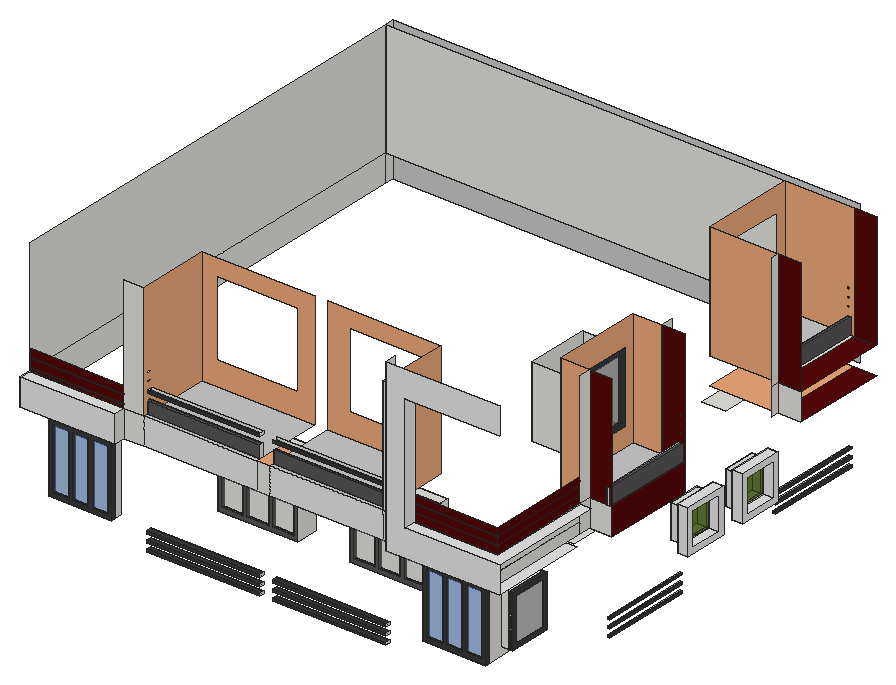
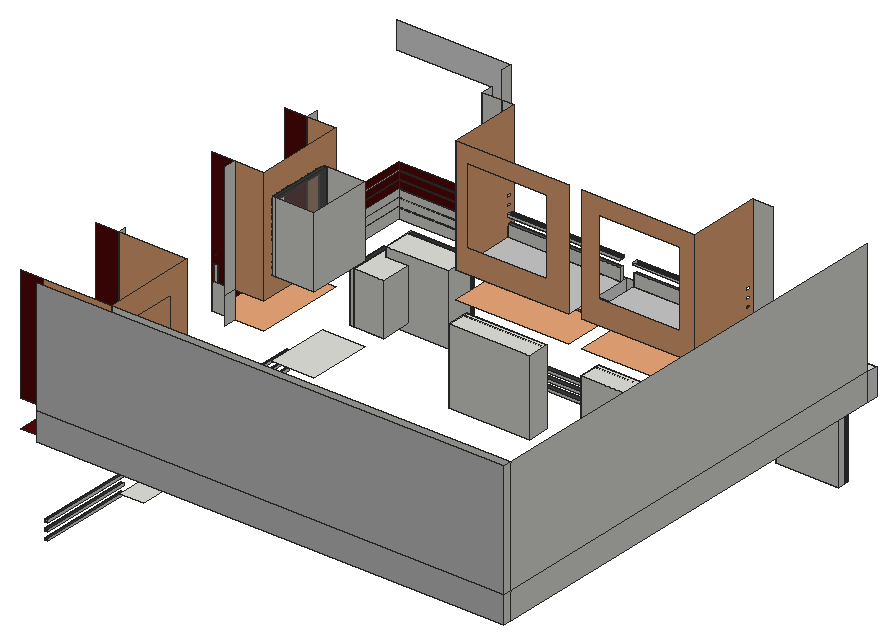
# SketchUp Ruby script. Lengths in inches.
U = 1.inch
M = Sketchup.active_model
def pt(a) = Geom::Point3d.new(a.map { |v| v * U })
def face(e, loops, mat)
  f = e.add_face(loops[0].map { |a| pt(a) })
  loops[1..].each { |l| e.add_face(l.map { |a| pt(a) }).erase! }
  f.material = f.back_material = mat if mat
  f
end
# faces: each face lists its corners as indices into pts; further lists are holes
def faces(e, pts, list, mat = nil) = list.each { |f| face(e, (f[0].is_a?(Array) ? f : [f]).map { |l| l.map { |i| pts[i] } }, mat) }
# xy, xz, yz: faces in a plane at the given z, y or x. An outline is a flat list of corners, or four numbers for a rectangle; further outlines are holes
def ring(l) = l.size == 4 ? [[l[0], l[1]], [l[2], l[1]], [l[2], l[3]], [l[0], l[3]]] : l.each_slice(2).to_a
def flat(e, list, mat, &to3) = list.each { |f| face(e, (f[0].is_a?(Array) ? f : [f]).map { |l| ring(l).map { |u, v| to3.(u, v) } }, mat) }
def xy(e, z, list, mat = nil) = flat(e, list, mat) { |x, y| [x, y, z] }
def xz(e, y, list, mat = nil) = flat(e, list, mat) { |x, z| [x, y, z] }
def yz(e, x, list, mat = nil) = flat(e, list, mat) { |y, z| [x, y, z] }
def lines(e, pts, list) = list.each { |a, b| e.add_line(pt(pts[a]), pt(pts[b])) }
# prism: a flat outline (further loops are holes) pulled along v
def prism(e, loops, v, mat = nil)
  f = face(e, loops, mat); d = Geom::Vector3d.new(v.map { |x| x * U })
  f.pushpull(f.normal.samedirection?(d) ? d.length : -d.length)
end
def box(e, o, s, mat = nil) = prism(e, [[o, [o[0] + s[0], o[1], o[2]], [o[0] + s[0], o[1] + s[1], o[2]], [o[0], o[1] + s[1], o[2]]]], [0, 0, s[2]], mat)
def at(x, y, z, deg = 0) = Geom::Transformation.translation(pt([x, y, z])) * Geom::Transformation.rotation(ORIGIN, Z_AXIS, deg.degrees)
def axes(o, x, y, z) = Geom::Transformation.new([*x, 0, *y, 0, *z, 0, *pt(o).to_a, 1])
def part(name) = M.definitions.add(name)
# library, detail: a bought-in or finely detailed component or shape, given as its bounding box
def library(name, o, s) = part(name).tap { |d| box(d.entities, o, s) }
def detail(e, o, s) = box(e.add_group.entities, o, s)
def put(e, d, t, mat = nil) = e.add_instance(d, t).tap { |i| i.material = mat if mat }
def group(e, t, mat = nil) = e.add_group.tap { |g| g.transformation = t; g.material = mat if mat }.entities
root = M.entities
M.materials.add("Generic").color = [86, 8, 8]
M.materials.add("Generic\#1").color = [236, 168, 122]
M.materials.add("Generic\#4").color = [201, 201, 201]
M.materials.add("Generic\#5").color = [230, 230, 230]
M.materials.add("[Color M06]").color = [86, 86, 86]
M.materials.add("[Color M07]").color = [58, 58, 58]
M.materials.add("[Mirror 01]").color = [185, 185, 185]
M.materials.add("[Mirror 02]1").color = [226, 226, 226]
M.materials["[Mirror 02]1"].alpha = 0.26
M.materials.add("[Translucent Glass Blue]").color = [100, 149, 237]
M.materials["[Translucent Glass Blue]"].alpha = 0.5
M.materials.add("[Translucent Glass Dark Green]").color = [62, 91, 5]
M.materials["[Translucent Glass Dark Green]"].alpha = 0.5
M.materials.add("[Translucent Glass Gray]").color = [127, 127, 127]
M.materials["[Translucent Glass Gray]"].alpha = 0.35
c1 = part("Group\#4")
xy(c1.entities,0,[[0,0,117.75,6]],"[Color M06]")
xy(c1.entities,6.37,[[6.37,0,37.125,3],[43.5,0,74.25,3],[80.625,0,111.38,3]],"[Color M06]")
xy(c1.entities,103.75,[[6.37,0,37.125,3],[43.5,0,74.25,3],[80.625,0,111.38,3]],"[Color M06]")
xy(c1.entities,110.125,[[0,0,117.75,6]],"[Color M06]")
xz(c1.entities,0,[[[0,0,117.75,110.125],[6.37,6.37,37.125,103.75],[80.625,6.37,111.38,103.75],[43.5,6.37,74.25,103.75]]],"[Color M06]")
xz(c1.entities,3,[[6.37,6.37,37.125,103.75],[43.5,6.37,74.25,103.75],[80.625,6.37,111.38,103.75]],"[Mirror 02]1")
xz(c1.entities,6,[[0,0,117.75,110.125]])
yz(c1.entities,0,[[0,0,6,110.125]],"[Color M06]")
yz(c1.entities,6.37,[[0,6.37,3,103.75]],"[Color M06]")
yz(c1.entities,37.125,[[0,6.37,3,103.75]],"[Color M06]")
yz(c1.entities,43.5,[[0,6.37,3,103.75]],"[Color M06]")
yz(c1.entities,74.25,[[0,6.37,3,103.75]],"[Color M06]")
yz(c1.entities,80.625,[[0,6.37,3,103.75]],"[Color M06]")
yz(c1.entities,111.38,[[0,6.37,3,103.75]],"[Color M06]")
yz(c1.entities,117.75,[[0,0,6,110.125]],"[Color M06]")
c2 = part("Group\#2")
xy(c2.entities,0,[[0,0,91.6875,6]],"[Color M07]")
xy(c2.entities,6.1,[[6.1,0,28.53,3],[34.63,0,57.06,3],[63.16,0,85.59,3]],"[Color M07]")
xy(c2.entities,95.34,[[6.1,0,28.53,3],[34.63,0,57.06,3],[63.16,0,85.59,3]],"[Color M07]")
xy(c2.entities,101.4375,[[0,0,91.6875,6]],"[Color M07]")
xz(c2.entities,0,[[[0,0,91.6875,101.4375],[34.63,6.1,57.06,95.34],[63.16,6.1,85.59,95.34],[6.1,6.1,28.53,95.34]]],"[Color M07]")
xz(c2.entities,3,[[6.1,6.1,28.53,95.34],[34.63,6.1,57.06,95.34],[63.16,6.1,85.59,95.34]],"[Translucent Glass Blue]")
xz(c2.entities,6,[[0,0,91.6875,101.4375]])
yz(c2.entities,0,[[0,0,6,101.4375]],"[Color M07]")
yz(c2.entities,6.1,[[0,6.1,3,95.34]],"[Color M07]")
yz(c2.entities,28.53,[[0,6.1,3,95.34]],"[Color M07]")
yz(c2.entities,34.63,[[0,6.1,3,95.34]],"[Color M07]")
yz(c2.entities,57.06,[[0,6.1,3,95.34]],"[Color M07]")
yz(c2.entities,63.16,[[0,6.1,3,95.34]],"[Color M07]")
yz(c2.entities,85.59,[[0,6.1,3,95.34]],"[Color M07]")
yz(c2.entities,91.6875,[[0,0,6,101.4375]],"[Color M07]")
c3 = part("Group\#3")
xy(c3.entities,0,[[0,0,6,62.6875]],"[Color M07]")
xy(c3.entities,6.1,[[3,6.1,6,56.59]],"[Color M07]")
xy(c3.entities,69.52,[[3,6.1,6,56.59]],"[Color M07]")
xy(c3.entities,75.625,[[0,0,6,62.6875]],"[Color M07]")
xz(c3.entities,0,[[0,0,6,75.625]],"[Color M07]")
xz(c3.entities,6.1,[[3,6.1,6,69.52]],"[Color M07]")
xz(c3.entities,56.59,[[3,6.1,6,69.52]],"[Color M07]")
xz(c3.entities,62.6875,[[0,0,6,75.625]],"[Color M07]")
yz(c3.entities,0,[[0,0,62.6875,75.625]])
yz(c3.entities,3,[[6.1,6.1,56.59,69.52]],"[Mirror 01]")
yz(c3.entities,6,[[[0,0,62.6875,75.625],[6.1,6.1,56.59,69.52]]],"[Color M07]")
c4 = part("Group\#1")
box(c4.entities,[0,0,0],[3,48.3125,48.3125],"[Translucent Glass Dark Green]")
c5 = library("Tlon Light 450 Ceiling 152 006",[-8.86,-8.86,-3.78],[17.72,17.72,3.56])
c6 = part("Group\#5")
xy(c6.entities,0,[[0,0,6,92.0625]],"[Color M07]")
xy(c6.entities,6.58,[[3,6.58,6,85.48]],"[Color M07]")
xy(c6.entities,96.73,[[3,6.58,6,85.48]],"[Color M07]")
xy(c6.entities,103.3125,[[0,0,6,92.0625]],"[Color M07]")
xz(c6.entities,0,[[0,0,6,103.3125]],"[Color M07]")
xz(c6.entities,6.58,[[3,6.58,6,96.73]],"[Color M07]")
xz(c6.entities,85.48,[[3,6.58,6,96.73]],"[Color M07]")
xz(c6.entities,92.0625,[[0,0,6,103.3125]],"[Color M07]")
yz(c6.entities,0,[[0,0,92.0625,103.3125]],"[Translucent Glass Gray]")
yz(c6.entities,3,[[6.58,6.58,85.48,96.73]],"[Translucent Glass Gray]")
yz(c6.entities,6,[[[0,0,92.0625,103.3125],[6.58,6.58,85.48,96.73]]],"[Color M07]")
xy(root,442.38,[[183.5625,118.5,347.9375,125.9375]],"[Color M07]")
xy(root,442.82,[[367.1875,118.5,531.5625,125.9375]],"[Color M07]")
xy(root,446.19,[[183.5625,118.5,347.9375,125.9375]],"[Color M07]")
xy(root,446.63,[[367.1875,118.5,531.5625,125.9375]],"[Color M07]")
xy(root,449.49,[[691.43,624.8125,695.61,762.8125]],"[Color M07]")
xy(root,449.67,[[724.45,281.625,727.82,413.625]],"[Color M07]")
xy(root,452.79,[[724.45,281.625,727.82,413.625]],"[Color M07]")
xy(root,452.8,[[691.43,624.8125,695.61,762.8125]],"[Color M07]")
xy(root,454.38,[[183.5625,118.5,347.9375,125.9375]],"[Color M07]")
xy(root,454.82,[[367.1875,118.5,531.5625,125.9375]],"[Color M07]")
xy(root,458.19,[[183.5625,118.5,347.9375,125.9375]],"[Color M07]")
xy(root,458.63,[[367.1875,118.5,531.5625,125.9375]],"[Color M07]")
xy(root,460.21,[[205.67,219.4375,323.42,251.5625],[397.99,219.4375,515.74,251.5625]])
xy(root,461.54,[[691.43,624.8125,695.61,762.8125]],"[Color M07]")
xy(root,461.67,[[724.45,281.625,727.82,413.625]],"[Color M07]")
xy(root,464.79,[[724.45,281.625,727.82,413.625]],"[Color M07]")
xy(root,464.85,[[691.43,624.8125,695.61,762.8125]],"[Color M07]")
xy(root,466.73,[[183.5625,118.5,347.9375,125.9375]],"[Color M07]")
xy(root,466.82,[[367.1875,118.5,531.5625,125.9375]],"[Color M07]")
xy(root,468.8,[[44.83,113.625,136.51,130.0625]])
xy(root,470.54,[[183.5625,118.5,347.9375,125.9375]],"[Color M07]")
xy(root,470.63,[[367.1875,118.5,531.5625,125.9375]],"[Color M07]")
xy(root,471.43,[[589.83,113.625,681.51,159.375]])
xy(root,473.54,[[691.43,624.8125,695.61,762.8125]],"[Color M07]")
xy(root,473.55,[[724.45,281.625,727.82,413.625]],"[Color M07]")
xy(root,476.68,[[724.45,281.625,727.82,413.625]],"[Color M07]")
xy(root,476.85,[[691.43,624.8125,695.61,762.8125]],"[Color M07]")
xy(root,480.05,[[698.4375,441.62,713.5625,506.43],[698.4375,541.56,713.5625,606.36]],"Generic\#5")
xy(root,483.99,[[648.625,141.33,698.4375,204.02]])
xy(root,488.3,[[681.875,449.87,698.4375,498.18],[681.875,549.8,698.4375,598.12]])
xy(root,488.3,[[698.4375,449.87,713.5625,498.18],[698.4375,549.8,713.5625,598.12]],"Generic\#5")
xy(root,536.61,[[681.875,449.87,698.4375,498.18],[681.875,549.8,698.4375,598.12]])
xy(root,536.61,[[698.4375,449.87,713.5625,498.18],[698.4375,549.8,713.5625,598.12]],"Generic\#5")
xy(root,536.98,[[594.5625,306.16,656.0625,398.23]])
xy(root,537.15,[[563.75,654.65,598.75,746.71]])
xy(root,544.86,[[698.4375,441.62,713.5625,506.43],[698.4375,541.56,713.5625,606.36]],"Generic\#5")
xy(root,559.61,[[648.625,141.33,698.4375,204.02]])
xy(root,570.24,[[44.83,113.625,136.51,130.0625]])
xy(root,570.34,[[205.67,219.4375,323.42,251.5625],[397.99,219.4375,515.74,251.5625]])
xy(root,572.86,[[589.83,113.625,681.51,159.375]])
xy(root,582.625,[[698.4375,624.8125,731.4375,762.8125]],"Generic")
xy(root,582.625,[[183.5625,113.625,347.9375,219.4375],[367.1875,113.625,531.5625,219.4375],[656.0625,281.625,731.4375,413.625],[598.75,624.8125,698.4375,762.8125]],"Generic\#1")
xy(root,582.625,[[16.6875,96.5625,154.5,113.625],[549.5625,96.5625,549.5625,113.625,698.4375,113.625,698.4375,238.3125,715.125,238.3125,715.125,96.5625]],"Generic\#5")
xy(root,621.9375,[[183.5625,119.625,347.9375,123.625],[367.1875,119.625,531.5625,123.625],[723.5625,281.625,728.4375,413.625],[689.1875,624.8125,693.6875,762.8125],[693.6875,624.8125,698.4375,762.8125]])
xy(root,621.9375,[[728.4375,281.625,731.4375,413.625],[698.4375,624.8125,731.4375,762.8125]],"Generic")
xy(root,621.9375,[[183.5625,113.625,347.9375,119.625],[367.1875,113.625,531.5625,119.625],[183.5625,123.625,347.9375,219.4375],[367.1875,123.625,531.5625,219.4375],[656.0625,281.625,723.5625,413.625],
  [598.75,624.8125,689.1875,762.8125]],"Generic\#4")
xy(root,621.9375,[[16.6875,96.5625,154.5,113.625],[577.6875,96.5625,715.125,96.5625,715.125,263.625,698.4375,263.625,698.4375,113.625,577.6875,113.625]],"Generic\#5")
xy(root,626.9375,[[16.6875,113.625,154.5,113.92]])
xy(root,627.9375,[[16.6875,113.625,154.5,113.92]])
xy(root,633.58,[[577.6875,113.625,698.4375,113.92],[698.14,113.92,698.4375,263.625]])
xy(root,634.58,[[577.6875,113.625,698.4375,113.92],[698.14,113.92,698.4375,263.625]])
xy(root,639.4375,[[16.6875,113.625,154.5,113.92]])
xy(root,639.9375,[[183.5625,119.625,347.9375,123.625],[367.1875,119.625,531.5625,123.625]],"[Color M06]")
xy(root,640.4375,[[16.6875,113.625,154.5,113.92]])
xy(root,645.53,[[577.6875,113.625,698.4375,113.92],[698.25,113.92,698.4375,263.625]])
xy(root,645.9375,[[723.5625,281.625,728.4375,413.625],[689.1875,624.8125,693.6875,762.8125]],"[Color M06]")
xy(root,646.53,[[577.6875,113.625,698.4375,113.92],[698.25,113.92,698.4375,263.625]])
xy(root,648.98,[[594.5625,306.16,656.0625,398.23]])
xy(root,650,[[367.1875,118.5,531.5625,125.9375]],"[Color M07]")
xy(root,650.73,[[183.5625,118.5,347.9375,125.9375]],"[Color M07]")
xz(root,96.5625,[[16.6875,582.625,154.5,621.9375],[549.5625,582.625,715.125,582.625,715.125,621.9375,577.6875,621.9375,577.6875,789.9375,715.125,789.9375,715.125,829.25,549.5625,829.25]],"Generic\#5")
xz(root,113.625,[[16.6875,582.625,154.5,589.4375],[154.5,582.625,183.4375,621.9375],[347.9375,582.625,367.1875,621.9375],[531.6875,582.625,549.5625,621.9375],[549.5625,582.625,549.5625,621.9375,577.6875,621.9375,577.6875,621.64,698.4375,621.64,698.4375,610.69,577.6875,610.69,577.6875,609.69,698.4375,609.69,698.4375,598.74,577.6875,598.74,577.6875,597.74,698.4375,597.74,698.4375,582.625],
  [16.6875,589.4375,154.5,590.4375],[16.6875,590.4375,154.5,601.9375],[577.6875,597.74,698.4375,598.74],[16.6875,601.9375,154.5,602.9375],[16.6875,602.9375,154.5,614.4375],
  [577.6875,609.69,698.4375,610.69],[16.6875,614.4375,154.5,615.4375],[16.6875,615.4375,154.5,621.9375],[577.6875,621.64,698.4375,621.9375],[154.5,621.9375,183.4375,789.9375],
  [183.4375,621.9375,183.5625,789.9375],[531.5625,621.9375,531.6875,789.9375],[531.6875,621.9375,549.5625,789.9375],[549.5625,621.9375,577.6875,789.9375]])
xz(root,113.625,[[16.6875,621.9375,154.5,626.9375],[577.6875,621.9375,698.4375,633.58],[16.6875,627.9375,154.5,639.4375],[577.6875,634.58,698.4375,645.53],[16.6875,640.4375,154.5,651.9375],
  [577.6875,646.53,698.4375,657.48]],"Generic")
xz(root,113.625,[[183.4375,582.625,347.9375,621.9375],[367.1875,582.625,531.6875,621.9375]],"Generic\#5")
xz(root,113.92,[[16.6875,626.9375,154.5,627.9375],[577.6875,633.58,698.14,634.58],[16.6875,639.4375,154.5,640.4375],[577.6875,645.53,698.25,646.53]])
xz(root,118.5,[[183.5625,442.38,347.9375,446.19],[367.1875,442.82,531.5625,446.63],[183.5625,454.38,347.9375,458.19],[367.1875,454.82,531.5625,458.63],[183.5625,466.73,347.9375,470.54],
  [367.1875,466.82,531.5625,470.63],[367.1875,650,531.5625,653.82],[183.5625,650.73,347.9375,654.54]],"[Color M07]")
xz(root,119.625,[[183.5625,621.9375,347.9375,639.9375],[367.1875,621.9375,531.5625,639.9375]],"[Color M06]")
xz(root,123.625,[[183.5625,621.9375,347.9375,639.9375],[367.1875,621.9375,531.5625,639.9375]])
xz(root,125.9375,[[183.5625,442.38,347.9375,446.19],[367.1875,442.82,531.5625,446.63],[183.5625,454.38,347.9375,458.19],[367.1875,454.82,531.5625,458.63],[183.5625,466.73,347.9375,470.54],
  [367.1875,466.82,531.5625,470.63],[367.1875,650,531.5625,653.82],[183.5625,650.73,347.9375,654.54]])
xz(root,130.0625,[[44.83,468.8,136.51,570.24]])
xz(root,141.33,[[648.625,483.99,698.4375,559.61]])
xz(root,159.375,[[589.83,471.43,681.51,572.86]])
xz(root,204.02,[[648.625,483.99,698.4375,559.61]])
xz(root,219.4375,[[[183.5625,621.9375,347.9375,789.9375],[205.11,656.21,322.86,766.34]],[[367.1875,621.9375,531.5625,789.9375],[397.99,656.21,515.74,766.34]]],"Generic\#1")
xz(root,251.5625,[[205.67,460.21,323.42,570.34],[397.99,460.21,515.74,570.34]])
xz(root,263.625,[[698.14,633.58,698.4375,634.58],[698.25,645.53,698.4375,646.53]])
xz(root,281.625,[[698.4375,582.625,731.4375,621.9375],[723.5625,621.9375,728.4375,645.9375]])
xz(root,281.625,[[[698.4375,621.9375,698.4375,789.9375,731.4375,789.9375,731.4375,621.9375,728.4375,621.9375,728.4375,645.9375,723.5625,645.9375,723.5625,621.9375],[723.95,680.79,727.32,683.92],[723.95,668.79,727.32,671.92],[723.95,656.79,727.32,659.92]]],"Generic")
xz(root,281.625,[[656.0625,621.9375,698.4375,789.9375]],"Generic\#1")
xz(root,306.16,[[594.5625,648.98,656.0625,752.29]])
xz(root,398.23,[[594.5625,648.98,656.0625,752.29]])
xz(root,413.625,[[724.45,449.67,727.82,452.79],[724.45,461.67,727.82,464.79],[724.45,473.55,727.82,476.68],[698.4375,582.625,731.4375,621.9375],[723.5625,621.9375,728.4375,645.9375]])
xz(root,413.625,[[[698.4375,621.9375,723.5625,621.9375,723.5625,645.9375,728.4375,645.9375,728.4375,621.9375,731.4375,621.9375,731.4375,789.9375,698.4375,789.9375],[723.95,656.79,727.32,659.92],[723.95,668.79,727.32,671.92],[723.95,680.79,727.32,683.92]]],"Generic")
xz(root,413.625,[[656.0625,621.9375,698.4375,789.9375]],"Generic\#1")
xz(root,441.62,[[698.4375,480.05,713.5625,544.86]],"Generic\#5")
xz(root,449.87,[[681.875,488.3,698.4375,536.61]])
xz(root,449.87,[[698.4375,488.3,713.5625,536.61]],"Generic\#5")
xz(root,498.18,[[681.875,488.3,698.4375,536.61]])
xz(root,498.18,[[698.4375,488.3,713.5625,536.61]],"Generic\#5")
xz(root,506.43,[[698.4375,480.05,713.5625,544.86]],"Generic\#5")
xz(root,541.56,[[698.4375,480.05,713.5625,544.86]],"Generic\#5")
xz(root,549.8,[[681.875,488.3,698.4375,536.61]])
xz(root,549.8,[[698.4375,488.3,713.5625,536.61]],"Generic\#5")
xz(root,598.12,[[681.875,488.3,698.4375,536.61]])
xz(root,598.12,[[698.4375,488.3,713.5625,536.61]],"Generic\#5")
xz(root,606.36,[[698.4375,480.05,713.5625,544.86]],"Generic\#5")
xz(root,624.8125,[[698.4375,582.625,731.4375,621.9375],[689.1875,621.9375,693.6875,645.9375]])
xz(root,624.8125,[[698.4375,621.9375,731.4375,789.9375]],"Generic")
xz(root,624.8125,[[[598.75,621.9375,598.75,789.9375,698.4375,789.9375,698.4375,621.9375,693.6875,621.9375,693.6875,645.9375,689.1875,645.9375,689.1875,621.9375],[688.37,680.8125,692.56,684.125],[688.37,668.8125,692.56,672.125],[689.08,656.83,693.27,660.15]]],"Generic\#1")
xz(root,762.8125,[[691.43,449.49,695.61,452.8],[691.43,461.54,695.61,464.85],[691.43,473.54,695.61,476.85],[16.6875,621.9375,598.75,789.9375],[689.1875,621.9375,693.6875,645.9375]])
xz(root,762.8125,[[698.4375,621.9375,731.4375,789.9375]],"Generic")
xz(root,762.8125,[[[598.75,621.9375,689.1875,621.9375,689.1875,645.9375,693.6875,645.9375,693.6875,621.9375,698.4375,621.9375,698.4375,789.9375,598.75,789.9375],[689.08,656.83,693.27,660.15],[688.37,668.8125,692.56,672.125],[688.37,680.8125,692.56,684.125]]],"Generic\#1")
xz(root,774.8125,[[16.6875,582.625,698.4375,621.9375],[16.6875,621.9375,698.4375,789.9375]],"Generic\#4")
yz(root,16.6875,[[113.625,582.625,762.8125,621.9375],[762.8125,582.625,774.8125,621.9375],[113.625,621.9375,113.625,626.9375,113.92,626.9375,113.92,627.9375,113.625,627.9375,113.625,639.4375,113.92,639.4375,113.92,640.4375,113.625,640.4375,113.625,651.9375,113.92,651.9375,113.92,652.9375,113.625,652.9375,113.625,664.4375,113.92,664.4375,113.92,665.4375,113.625,665.4375,113.625,676.9375,113.92,676.9375,113.92,677.9375,113.625,677.9375,113.625,689.4375,113.92,689.4375,113.92,690.4375,113.625,690.4375,113.625,701.9375,113.92,701.9375,113.92,702.9375,113.625,702.9375,113.625,714.4375,113.92,714.4375,113.92,715.4375,113.625,715.4375,113.625,726.9375,113.92,726.9375,113.92,727.9375,113.625,727.9375,113.625,739.4375,113.92,739.4375,113.92,740.4375,113.625,740.4375,113.625,751.9375,113.92,751.9375,113.92,752.9375,113.625,752.9375,113.625,764.4375,113.92,764.4375,113.92,765.4375,113.625,765.4375,113.625,776.9375,113.92,776.9375,113.92,777.9375,113.625,777.9375,113.625,789.9375,762.8125,789.9375,762.8125,621.9375],[762.8125,621.9375,774.8125,789.9375]])
yz(root,16.6875,[[96.5625,582.625,113.625,621.9375]],"Generic\#5")
yz(root,44.83,[[113.625,468.8,130.0625,570.24]])
yz(root,136.51,[[113.625,468.8,130.0625,570.24]])
yz(root,154.5,[[96.5625,582.625,113.625,621.9375],[113.625,626.9375,113.92,627.9375],[113.625,639.4375,113.92,640.4375]])
yz(root,183.5625,[[119.625,621.9375,123.625,639.9375]])
yz(root,183.5625,[[[113.625,621.9375,119.625,621.9375,119.625,639.9375,123.625,639.9375,123.625,621.9375,219.4375,621.9375,219.4375,789.9375,113.625,789.9375],[118.5,674.73,125.9375,678.54],[118.5,662.73,125.9375,666.54],[118.5,650.73,125.9375,654.54]]],"Generic\#1")
yz(root,205.67,[[219.4375,460.21,251.5625,570.34]])
yz(root,323.42,[[219.4375,460.21,251.5625,570.34]])
yz(root,347.9375,[[118.5,442.38,125.9375,446.19],[118.5,454.38,125.9375,458.19],[118.5,466.73,125.9375,470.54],[119.625,621.9375,123.625,639.9375],[118.5,650.73,125.9375,654.54]])
yz(root,367.1875,[[119.625,621.9375,123.625,639.9375]])
yz(root,397.99,[[219.4375,460.21,251.5625,570.34]])
yz(root,515.74,[[219.4375,460.21,251.5625,570.34]])
yz(root,531.5625,[[118.5,442.82,125.9375,446.63],[118.5,454.82,125.9375,458.63],[118.5,466.82,125.9375,470.63],[119.625,621.9375,123.625,639.9375],[118.5,650,125.9375,653.82]])
yz(root,531.5625,[[[113.625,621.9375,113.625,789.9375,219.4375,789.9375,219.4375,621.9375,123.625,621.9375,123.625,639.9375,119.625,639.9375,119.625,621.9375],[118.5,674,125.9375,677.82],[118.5,662,125.9375,665.82],[118.5,650,125.9375,653.82]]],"Generic\#1")
yz(root,549.5625,[[96.5625,582.625,113.625,621.9375],[96.5625,621.9375,113.625,829.25]])
yz(root,577.6875,[[113.625,633.58,113.92,634.58],[113.625,645.53,113.92,646.53]])
yz(root,577.6875,[[96.5625,621.9375,113.625,789.9375]],"Generic\#5")
yz(root,589.83,[[113.625,471.43,159.375,572.86]])
yz(root,594.5625,[[306.16,648.98,398.23,752.29]])
yz(root,598.75,[[[624.8125,621.9375,762.8125,789.9375],[654.65,652.65,746.71,755.96]]],"Generic\#1")
yz(root,648.625,[[141.33,483.99,204.02,559.61]])
yz(root,656.0625,[[[281.625,621.9375,413.625,789.9375],[306.16,648.98,398.23,752.29]]],"Generic\#1")
yz(root,681.51,[[113.625,471.43,159.375,572.86]])
yz(root,681.875,[[449.87,488.3,498.18,536.61],[549.8,488.3,598.12,536.61]])
yz(root,689.1875,[[624.8125,621.9375,762.8125,645.9375]])
yz(root,691.43,[[624.8125,449.49,762.8125,452.8],[624.8125,461.54,762.8125,464.85],[624.8125,473.54,762.8125,476.85]])
yz(root,693.6875,[[624.8125,621.9375,762.8125,645.9375]],"[Color M06]")
yz(root,695.61,[[624.8125,449.49,762.8125,452.8],[624.8125,461.54,762.8125,464.85],[624.8125,473.54,762.8125,476.85]],"[Color M07]")
yz(root,698.14,[[113.92,633.58,263.625,634.58]])
yz(root,698.25,[[113.92,645.53,263.625,646.53]])
yz(root,698.4375,[[[441.62,480.05,506.43,544.86],[449.87,488.3,498.18,536.61]],[[541.56,480.05,606.36,544.86],[549.8,488.3,598.12,536.61]],[113.625,582.625,263.625,598.4],[263.625,582.625,281.625,621.9375],[413.625,582.625,431.625,621.9375],
  [612.8125,582.625,624.8125,621.9375],[113.625,598.4,263.625,599.4],[113.625,599.4,263.625,610.3],[113.625,610.3,263.625,611.3],[113.625,611.3,263.625,621.9375],
  [263.625,621.9375,281.625,789.9375],[413.625,621.9375,431.625,789.9375],[612.8125,621.9375,624.8125,789.9375]])
yz(root,698.4375,[[113.625,621.9375,263.625,633.58],[113.625,634.58,263.625,645.53],[113.625,646.53,263.625,657.48]],"Generic")
yz(root,713.5625,[[[441.62,480.05,506.43,544.86],[449.87,488.3,498.18,536.61]],[[541.56,480.05,606.36,544.86],[549.8,488.3,598.12,536.61]]],"Generic\#5")
yz(root,723.5625,[[281.625,621.9375,413.625,645.9375]])
yz(root,724.45,[[281.625,449.67,413.625,452.79],[281.625,461.67,413.625,464.79],[281.625,473.55,413.625,476.68]])
yz(root,727.82,[[281.625,449.67,413.625,452.79],[281.625,461.67,413.625,464.79],[281.625,473.55,413.625,476.68]],"[Color M07]")
yz(root,728.4375,[[281.625,621.9375,413.625,645.9375]],"[Color M06]")
yz(root,731.4375,[[281.625,582.625,413.625,621.9375]],"Generic")
p = [[531.5625,121.625,444.625],[367.1875,121.625,444.625],[531.5625,121.625,456.625],[367.1875,121.625,456.625],[531.5625,121.625,468.625],[367.1875,121.625,468.625],
  [347.9375,121.625,444.625],[183.5625,121.625,444.625],[347.9375,121.625,456.625],[183.5625,121.625,456.625],[347.9375,121.625,468.625],[183.5625,121.625,468.625],
  [693.8125,762.8125,450.625],[693.8125,624.8125,450.625],[693.8125,762.8125,462.625],[693.8125,624.8125,462.625],[693.8125,762.8125,474.625],[693.8125,624.8125,474.625],
  [726,413.625,450.625],[726,281.625,450.625],[726,413.625,462.625],[726,281.625,462.625],[726,413.625,474.625],[726,281.625,474.625]]
lines(root,p,[[0,1],[2,3],[4,5],[6,7],[8,9],[10,11],[12,13],[14,15],[16,17],[18,19],[20,21],[22,23]])
put(root,c1,at(397.99,219.4375,460.21))
put(root,c1,at(205.67,219.4375,460.21))
put(root,c2,at(44.83,113.625,468.8))
put(root,c2,at(589.83,113.625,471.43))
put(root,c3,at(692.4375,141.33,483.99))
put(root,c4,at(695.4375,549.8,488.3))
put(root,c4,at(695.4375,449.87,488.3))
put(root,c5,at(220.56,143.45,584.54))
put(root,c5,at(313.99,143.45,584.54))
put(root,c5,at(405.56,143.45,584.54))
put(root,c5,at(507.93,143.45,584.54))
put(root,c6,at(650.0625,306.16,648.98))
